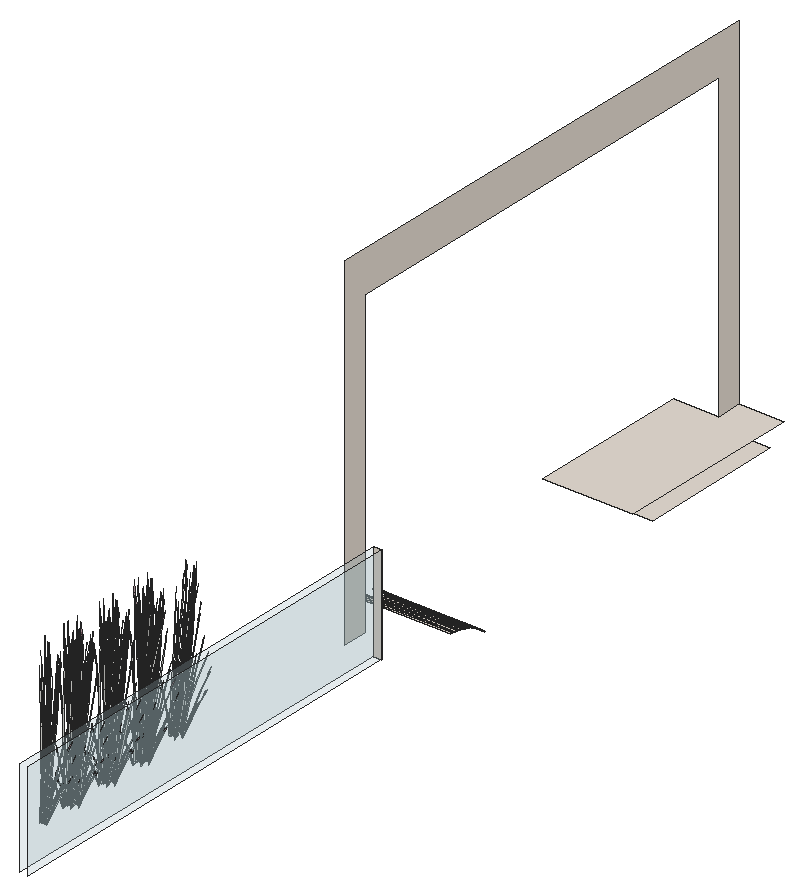
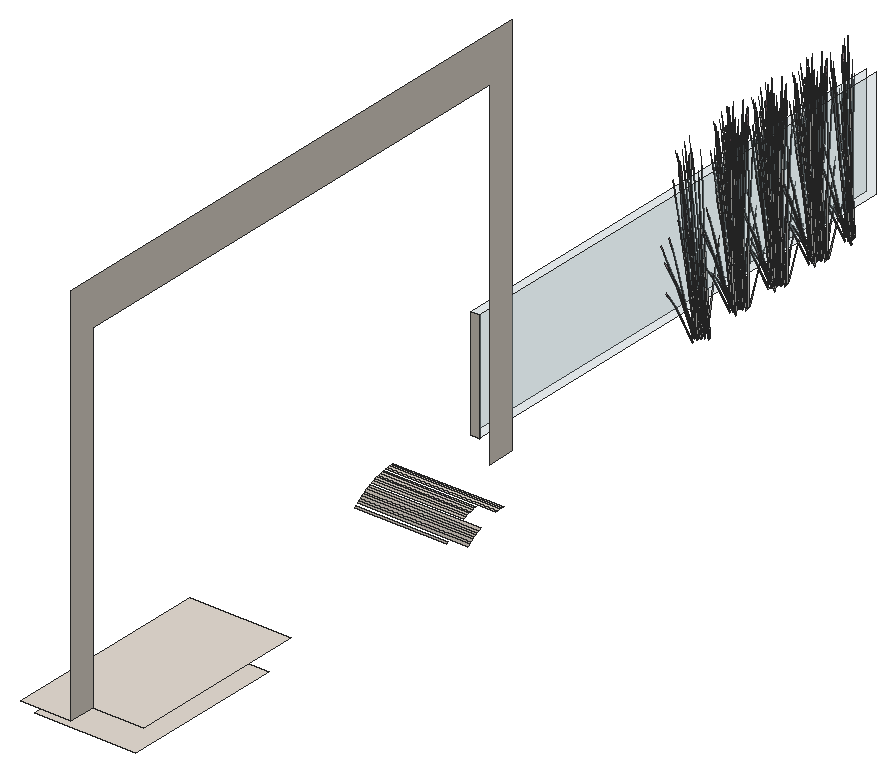
# SketchUp Ruby script. Lengths in inches.
U = 1.inch
M = Sketchup.active_model
def pt(a) = Geom::Point3d.new(a.map { |v| v * U })
def face(e, loops, mat)
  f = e.add_face(loops[0].map { |a| pt(a) })
  loops[1..].each { |l| e.add_face(l.map { |a| pt(a) }).erase! }
  f.material = f.back_material = mat if mat
  f
end
# faces: each face lists its corners as indices into pts; further lists are holes
def faces(e, pts, list, mat = nil) = list.each { |f| face(e, (f[0].is_a?(Array) ? f : [f]).map { |l| l.map { |i| pts[i] } }, mat) }
# xy, xz, yz: faces in a plane at the given z, y or x. An outline is a flat list of corners, or four numbers for a rectangle; further outlines are holes
def ring(l) = l.size == 4 ? [[l[0], l[1]], [l[2], l[1]], [l[2], l[3]], [l[0], l[3]]] : l.each_slice(2).to_a
def flat(e, list, mat, &to3) = list.each { |f| face(e, (f[0].is_a?(Array) ? f : [f]).map { |l| ring(l).map { |u, v| to3.(u, v) } }, mat) }
def xy(e, z, list, mat = nil) = flat(e, list, mat) { |x, y| [x, y, z] }
def xz(e, y, list, mat = nil) = flat(e, list, mat) { |x, z| [x, y, z] }
def yz(e, x, list, mat = nil) = flat(e, list, mat) { |y, z| [x, y, z] }
def lines(e, pts, list) = list.each { |a, b| e.add_line(pt(pts[a]), pt(pts[b])) }
# prism: a flat outline (further loops are holes) pulled along v
def prism(e, loops, v, mat = nil)
  f = face(e, loops, mat); d = Geom::Vector3d.new(v.map { |x| x * U })
  f.pushpull(f.normal.samedirection?(d) ? d.length : -d.length)
end
def box(e, o, s, mat = nil) = prism(e, [[o, [o[0] + s[0], o[1], o[2]], [o[0] + s[0], o[1] + s[1], o[2]], [o[0], o[1] + s[1], o[2]]]], [0, 0, s[2]], mat)
def at(x, y, z, deg = 0) = Geom::Transformation.translation(pt([x, y, z])) * Geom::Transformation.rotation(ORIGIN, Z_AXIS, deg.degrees)
def axes(o, x, y, z) = Geom::Transformation.new([*x, 0, *y, 0, *z, 0, *pt(o).to_a, 1])
def part(name) = M.definitions.add(name)
# library, detail: a bought-in or finely detailed component or shape, given as its bounding box
def library(name, o, s) = part(name).tap { |d| box(d.entities, o, s) }
def detail(e, o, s) = box(e.add_group.entities, o, s)
def put(e, d, t, mat = nil) = e.add_instance(d, t).tap { |i| i.material = mat if mat }
def group(e, t, mat = nil) = e.add_group.tap { |g| g.transformation = t; g.material = mat if mat }.entities
root = M.entities
M.materials.add("Glass_Safety_01").color = [204, 235, 244]
M.materials["Glass_Safety_01"].alpha = 0.25
M.materials.add("LightPink_Translucent").color = [144, 107, 117]
M.materials["LightPink_Translucent"].alpha = 0.75
M.materials.add("Marble_01_1K").color = [230, 221, 211]
c1 = part("blade")
p = [[2.15,0.21,22],[0,0.17,0],[0.09,0.45,0],[2.18,0.31,22],[2.29,0.31,22],[0.38,0.45,0],
  [2.48,0.24,33],[2.49,0.24,33],[2.48,0.22,33]]
faces(c1.entities,p,[[0,1,2,3],[4,5,2,3],[6,3,4,7],[8,0,3,6]])
c2 = part("seeds")
p = [[0.3,-0.1,1.38],[-0.01,-0.03,1.59],[-0.01,-0.03,0.03],[0.14,-0.07,-0.07],[0.29,-0.03,3],[0.15,0.01,3.11]]
faces(c2.entities,p,[[0,1,2,3],[1,0,4,5]],"LightPink_Translucent")
c3 = part("blade with seeds")
put(c3.entities,c1,at(0,0,0))
put(c3.entities,c2,axes([2.4,0.25,30.99],[1.5799,-0.05474,1.17369],[-0.12525,1.92788,0.29478],[-0.07173,-0.02425,1.56792]))
xy(root,258,[[321,336,354,390]],"Marble_01_1K")
xy(root,264,[[321,327,354,327,354,396,337.5,396,337.5,387,321,387]],"Marble_01_1K")
xz(root,216,[[348,264,351,300]],"Marble_01_1K")
yz(root,337.5,[[216,264,225,264,225,375,387,375,387,264,396,264,396,390,216,390]],"Marble_01_1K")
yz(root,348,[[54.05,264,216,300]],"Glass_Safety_01")
yz(root,351,[[54,264,216,300]],"Glass_Safety_01")
p = [[357,255.125,258.3],[357,255.69,257.81],[327,255.69,257.81],[327,255.125,258.3],[357,253.95,259.22],[357,254.54,258.77],
  [321,254.54,258.77],[321,253.95,259.22],[357,253.34,259.65],[321,253.34,259.65],[357,252.71,260.07],[321,252.71,260.07],
  [357,252.08,260.46],[321,252.08,260.46],[357,251.43,260.84],[321,251.43,260.84],[357,250.77,261.2],[321,250.77,261.2],
  [357,250.11,261.54],[321,250.11,261.54],[357,249.43,261.85],[321,249.43,261.85],[357,248.04,262.42],[357,248.74,262.15],
  [327,248.74,262.15],[327,248.04,262.42],[357,247.34,262.68],[327,247.34,262.68],[357,246.625,262.91],[327,246.625,262.91],
  [357,245.91,263.12],[327,245.91,263.12],[357,245.18,263.31],[327,245.18,263.31],[357,244.45,263.47],[327,244.45,263.47],
  [357,243.72,263.62],[327,243.72,263.62],[357,242.24,263.84],[357,242.98,263.74],[321,242.98,263.74],[321,242.24,263.84],
  [357,241.49,263.91],[321,241.49,263.91],[357,240.75,263.97],[321,240.75,263.97],[357,240,264],[321,240,264]]
faces(root,p,[[0,1,2,3],[4,5,6,7],[8,4,7,9],[10,8,9,11],[12,10,11,13],[14,12,13,15],[16,14,15,17],[18,16,17,19],
  [20,18,19,21],[22,23,24,25],[26,22,25,27],[28,26,27,29],[30,28,29,31],[32,30,31,33],[34,32,33,35],[36,34,35,37],
  [38,39,40,41],[42,38,41,43],[44,42,43,45],[46,44,45,47]],"Marble_01_1K")
put(root,c3,axes([336.35,109.73,266.4375],[0.37783,0.32657,0.13483],[-0.31516,0.36844,-0.38503],[-0.08772,0.04981,1.18024]))
put(root,c3,axes([336.35,93.3125,266.4375],[0.37783,0.32657,0.13483],[-0.31516,0.36844,-0.38503],[-0.08772,0.04981,1.18024]))
put(root,c3,axes([336.35,78.43,266.4375],[0.37783,0.32657,0.13483],[-0.31516,0.36844,-0.38503],[-0.08772,0.04981,1.18024]))
put(root,c3,axes([336.21,125.17,266.14],[-0.47569,-0.46784,-0.05709],[0.47598,-0.46812,0],[-0.01661,-0.01634,1.63492]))
put(root,c3,axes([336.21,109.33,266.14],[-0.47569,-0.46784,-0.05709],[0.47598,-0.46812,0],[-0.01661,-0.01634,1.63492]))
put(root,c3,axes([336.21,92.91,266.14],[-0.47569,-0.46784,-0.05709],[0.47598,-0.46812,0],[-0.01661,-0.01634,1.63492]))
put(root,c3,axes([336.34,125.33,266.53],[0.55535,-0.03355,0.41661],[0.05022,0.55698,-0.2005],[-0.09942,0.05645,1.33761]))
put(root,c3,axes([336.34,109.49,266.53],[0.55535,-0.03355,0.41661],[0.05022,0.55698,-0.2005],[-0.09942,0.05645,1.33761]))
put(root,c3,axes([336.34,93.07,266.53],[0.55535,-0.03355,0.41661],[0.05022,0.55698,-0.2005],[-0.09942,0.05645,1.33761]))
put(root,c3,axes([336.34,78.1875,266.53],[0.55535,-0.03355,0.41661],[0.05022,0.55698,-0.2005],[-0.09942,0.05645,1.33761]))
put(root,c3,axes([334.31,142.81,266.48],[0.57594,0.25935,-0.27094],[-0.27732,0.5474,-0.46562],[0.0181,0.1344,1.4872]))
put(root,c3,axes([336.47,126.61,266.17],[0.64025,0.17667,0.2864],[-0.16018,0.63149,-0.33981],[-0.10597,0.07904,1.53541]))
put(root,c3,axes([336.47,110.77,266.17],[0.64025,0.17667,0.2864],[-0.16018,0.63149,-0.33981],[-0.10597,0.07904,1.53541]))
put(root,c3,axes([336.47,94.35,266.17],[0.64025,0.17667,0.2864],[-0.16018,0.63149,-0.33981],[-0.10597,0.07904,1.53541]))
put(root,c3,axes([336.47,79.47,266.17],[0.64025,0.17667,0.2864],[-0.16018,0.63149,-0.33981],[-0.10597,0.07904,1.53541]))
put(root,c3,axes([335.54,121.77,265.39],[-0.08578,0.01958,1.6421],[-0.47437,-0.22044,-0.25086],[0.00796,-0.18387,0.2797]))
put(root,c3,axes([335.54,105.93,265.39],[-0.08578,0.01958,1.6421],[-0.47437,-0.22044,-0.25086],[0.00796,-0.18387,0.2797]))
put(root,c3,axes([335.54,89.51,265.39],[-0.08578,0.01958,1.6421],[-0.47437,-0.22044,-0.25086],[0.00796,-0.18387,0.2797]))
put(root,c3,axes([333.08,140.95,265.89],[0.47712,0.13449,-0.28847],[-0.12013,0.47362,0.28847],[0.09619,-0.05462,1.29413]))
put(root,c3,axes([336.75,126.58,266.31],[0.47863,-0.27177,0.46235],[0.28609,0.48733,0],[-0.10901,0.0619,1.46668]))
put(root,c3,axes([336.75,110.74,266.31],[0.47863,-0.27177,0.46235],[0.28609,0.48733,0],[-0.10901,0.0619,1.46668]))
put(root,c3,axes([336.75,94.32,266.31],[0.47863,-0.27177,0.46235],[0.28609,0.48733,0],[-0.10901,0.0619,1.46668]))
put(root,c3,axes([336.75,79.43,266.31],[0.47863,-0.27177,0.46235],[0.28609,0.48733,0],[-0.10901,0.0619,1.46668]))
put(root,c3,axes([334.41,140.375,266.41],[-0.14537,0.11002,1.33163],[-0.43536,-0.19256,-0.28638],[0.0807,-0.23948,0.56934]))
put(root,c3,axes([335.25,124.63,266.2],[0.22235,0.6078,0.42607],[-0.63531,0.21135,0.16719],[0.00776,-0.11168,1.47927]))
put(root,c3,axes([335.25,108.79,266.2],[0.22235,0.6078,0.42607],[-0.63531,0.21135,0.16719],[0.00776,-0.11168,1.47927]))
put(root,c3,axes([335.25,92.37,266.2],[0.22235,0.6078,0.42607],[-0.63531,0.21135,0.16719],[0.00776,-0.11168,1.47927]))
put(root,c3,axes([335.15,124.55,266.06],[0.24813,-0.48978,-0.41661],[0.51557,0.23571,0.2005],[0,-0.1129,1.33761]))
put(root,c3,axes([335.15,108.71,266.06],[0.24813,-0.48978,-0.41661],[0.51557,0.23571,0.2005],[0,-0.1129,1.33761]))
put(root,c3,axes([335.15,92.29,266.06],[0.24813,-0.48978,-0.41661],[0.51557,0.23571,0.2005],[0,-0.1129,1.33761]))
put(root,c3,axes([335.79,126.13,266.05],[-0.16686,-0.46861,0],[0.47648,-0.16411,0],[0,0,1.4375]))
put(root,c3,axes([335.79,110.29,266.05],[-0.16686,-0.46861,0],[0.47648,-0.16411,0],[0,0,1.4375]))
put(root,c3,axes([335.79,93.875,266.05],[-0.16686,-0.46861,0],[0.47648,-0.16411,0],[0,0,1.4375]))
put(root,c3,axes([335.18,127.12,265.39],[0.08277,-0.02958,1.6421],[0.49786,0.16279,-0.25086],[0.01456,0.18348,0.2797]))
put(root,c3,axes([335.18,111.28,265.39],[0.08277,-0.02958,1.6421],[0.49786,0.16279,-0.25086],[0.01456,0.18348,0.2797]))
put(root,c3,axes([335.18,94.86,265.39],[0.08277,-0.02958,1.6421],[0.49786,0.16279,-0.25086],[0.01456,0.18348,0.2797]))
put(root,c3,axes([335.18,79.98,265.39],[0.08277,-0.02958,1.6421],[0.49786,0.16279,-0.25086],[0.01456,0.18348,0.2797]))
put(root,c3,axes([335.56,142.93,266.31],[0,-0.54355,0.46235],[0.57217,0,0],[0,0.1238,1.46668]))
put(root,c3,axes([335.8,143.4375,265.88],[0,0.54355,-0.46235],[-0.57217,0,0],[0,0.1238,1.46668]))
put(root,c3,axes([332.97,140.73,265.88],[0.47863,-0.27177,-0.46235],[0.28609,0.48733,0],[0.10901,-0.0619,1.46668]))
put(root,c3,axes([333.93,142.08,266.4375],[0.09866,-0.48509,0.13483],[0.48202,0.0842,-0.38503],[0.08772,0.04981,1.18024]))
put(root,c3,axes([334.61,141.24,266.31],[-0.47863,-0.27177,0.46235],[0.28609,-0.48733,0],[0.10901,0.0619,1.46668]))
put(root,c3,axes([336.46,125.21,266.06],[-0.24813,0.48978,-0.41661],[-0.51557,-0.23571,0.2005],[0,0.1129,1.33761]))
put(root,c3,axes([336.46,109.37,266.06],[-0.24813,0.48978,-0.41661],[-0.51557,-0.23571,0.2005],[0,0.1129,1.33761]))
put(root,c3,axes([336.46,92.95,266.06],[-0.24813,0.48978,-0.41661],[-0.51557,-0.23571,0.2005],[0,0.1129,1.33761]))
put(root,c3,axes([336.46,78.0625,266.06],[-0.24813,0.48978,-0.41661],[-0.51557,-0.23571,0.2005],[0,0.1129,1.33761]))
put(root,c3,axes([334.2,144.07,266.03],[0.53691,-0.18442,-0.17877],[0.18866,0.53125,0.00007],[0.05927,-0.02038,1.61933]))
put(root,c3,axes([337.44,124.91,266.3],[-0.40181,-0.39593,0.16428],[0.40492,-0.38402,0.32672],[-0.04438,0.08086,1.49371]))
put(root,c3,axes([337.44,109.07,266.3],[-0.40181,-0.39593,0.16428],[0.40492,-0.38402,0.32672],[-0.04438,0.08086,1.49371]))
put(root,c3,axes([337.44,92.65,266.3],[-0.40181,-0.39593,0.16428],[0.40492,-0.38402,0.32672],[-0.04438,0.08086,1.49371]))
put(root,c3,axes([336.05,124.68,266.05],[0,-0.62892,0],[0.63949,0,0],[0,0,1.6711]))
put(root,c3,axes([336.05,108.84,266.05],[0,-0.62892,0],[0.63949,0,0],[0,0,1.6711]))
put(root,c3,axes([336.05,92.42,266.05],[0,-0.62892,0],[0.63949,0,0],[0,0,1.6711]))
put(root,c3,axes([335.46,124.79,266.27],[0.57623,0.26344,0.22409],[-0.27732,0.5474,0.46562],[0,-0.12618,1.49497]))
put(root,c3,axes([335.46,108.96,266.27],[0.57623,0.26344,0.22409],[-0.27732,0.5474,0.46562],[0,-0.12618,1.49497]))
put(root,c3,axes([335.46,92.54,266.27],[0.57623,0.26344,0.22409],[-0.27732,0.5474,0.46562],[0,-0.12618,1.49497]))
put(root,c3,axes([336.375,124.93,266.13],[0,0.62861,-0.05249],[-0.63949,0,0],[0,0.01975,1.67027]))
put(root,c3,axes([336.375,109.09,266.13],[0,0.62861,-0.05249],[-0.63949,0,0],[0,0.01975,1.67027]))
put(root,c3,axes([336.375,92.67,266.13],[0,0.62861,-0.05249],[-0.63949,0,0],[0,0.01975,1.67027]))
put(root,c3,axes([336.375,77.79,266.13],[0,0.62861,-0.05249],[-0.63949,0,0],[0,0.01975,1.67027]))
put(root,c3,axes([335.27,124.43,266.53],[-0.55535,0.03355,0.41661],[-0.05022,-0.55698,-0.2005],[0.09942,-0.05645,1.33761]))
put(root,c3,axes([335.27,108.59,266.53],[-0.55535,0.03355,0.41661],[-0.05022,-0.55698,-0.2005],[0.09942,-0.05645,1.33761]))
put(root,c3,axes([335.27,92.17,266.53],[-0.55535,0.03355,0.41661],[-0.05022,-0.55698,-0.2005],[0.09942,-0.05645,1.33761]))
put(root,c3,axes([334.21,142.5,266.06],[0.30722,0.45622,-0.41661],[-0.46535,0.32126,0.2005],[0.09942,0.05645,1.33761]))
put(root,c3,axes([335.02,123.47,266.3],[-0.14774,0.54019,0.16428],[-0.54062,-0.15287,0.32672],[0.09339,-0.00263,1.49371]))
put(root,c3,axes([335.02,107.63,266.3],[-0.14774,0.54019,0.16428],[-0.54062,-0.15287,0.32672],[0.09339,-0.00263,1.49371]))
put(root,c3,axes([335.02,91.21,266.3],[-0.14774,0.54019,0.16428],[-0.54062,-0.15287,0.32672],[0.09339,-0.00263,1.49371]))
put(root,c3,axes([336.07,126.15,266.13],[0.22235,0.62444,-0.05599],[-0.63531,0.21881,0],[0.00776,0.02181,1.60327]))
put(root,c3,axes([336.07,110.31,266.13],[0.22235,0.62444,-0.05599],[-0.63531,0.21881,0],[0.00776,0.02181,1.60327]))
put(root,c3,axes([336.07,93.89,266.13],[0.22235,0.62444,-0.05599],[-0.63531,0.21881,0],[0.00776,0.02181,1.60327]))
put(root,c3,axes([336.07,79,266.13],[0.22235,0.62444,-0.05599],[-0.63531,0.21881,0],[0.00776,0.02181,1.60327]))
put(root,c3,axes([334.05,144.4,266.41],[0.00902,-0.18018,1.33163],[0.43127,-0.20126,-0.28638],[0.13313,0.21566,0.56934]))
put(root,c3,axes([334.75,122.81,266.21],[-0.31974,-0.54466,0],[0.53494,-0.30375,-0.48057],[0.12184,-0.06918,1.52448]))
put(root,c3,axes([334.75,106.97,266.21],[-0.31974,-0.54466,0],[0.53494,-0.30375,-0.48057],[0.12184,-0.06918,1.52448]))
put(root,c3,axes([334.75,90.55,266.21],[-0.31974,-0.54466,0],[0.53494,-0.30375,-0.48057],[0.12184,-0.06918,1.52448]))
put(root,c3,axes([337.91,125.33,266.05],[-0.63917,-0.00435,-0.04634],[0,-0.60749,0.46507],[-0.02009,0.13829,1.47457]))
put(root,c3,axes([337.91,109.49,266.05],[-0.63917,-0.00435,-0.04634],[0,-0.60749,0.46507],[-0.02009,0.13829,1.47457]))
put(root,c3,axes([337.91,93.07,266.05],[-0.63917,-0.00435,-0.04634],[0,-0.60749,0.46507],[-0.02009,0.13829,1.47457]))
put(root,c3,axes([337.91,78.18,266.05],[-0.63917,-0.00435,-0.04634],[0,-0.60749,0.46507],[-0.02009,0.13829,1.47457]))
put(root,c3,axes([333.54,141.85,265.92],[0.34446,-0.40855,-0.58063],[0.42791,0.37046,-0.15239],[0.13803,-0.10191,1.28164]))
put(root,c3,axes([336.65,123.5,266.3],[-0.54955,0.14427,0.16428],[-0.1357,-0.53689,0.32672],[0.04901,0.07823,1.49371]))
put(root,c3,axes([336.65,107.66,266.3],[-0.54955,0.14427,0.16428],[-0.1357,-0.53689,0.32672],[0.04901,0.07823,1.49371]))
put(root,c3,axes([336.65,91.24,266.3],[-0.54955,0.14427,0.16428],[-0.1357,-0.53689,0.32672],[0.04901,0.07823,1.49371]))
put(root,c3,axes([336.09,105.65,266.58],[0.06561,0.31695,1.06958],[-0.36394,-0.17555,0.78586],[0.03916,-0.16229,0.23558]))
put(root,c3,axes([336.09,89.23,266.58],[0.06561,0.31695,1.06958],[-0.36394,-0.17555,0.78586],[0.03916,-0.16229,0.23558]))
put(root,c3,axes([335.05,141.48,265.89],[0.12013,0.47362,-0.28847],[-0.47712,0.13449,0.28847],[0.09619,0.05462,1.29413]))
put(root,c3,axes([335.95,143.03,266.21],[0.63949,0,0],[0,0.60749,-0.48057],[0,0.13836,1.52448]))
put(root,c3,axes([335.75,124.28,266.2],[-0.42403,0.49328,0.42607],[-0.50377,-0.43543,0.16719],[0.10223,-0.04923,1.47927]))
put(root,c3,axes([335.75,108.44,266.2],[-0.42403,0.49328,0.42607],[-0.50377,-0.43543,0.16719],[0.10223,-0.04923,1.47927]))
put(root,c3,axes([335.75,92.03,266.2],[-0.42403,0.49328,0.42607],[-0.50377,-0.43543,0.16719],[0.10223,-0.04923,1.47927]))
put(root,c3,axes([336.48,125.0625,266.0625],[0.35699,0.35109,0],[-0.35699,0.35109,0],[0,0,1.57621]))
put(root,c3,axes([336.48,109.22,266.0625],[0.35699,0.35109,0],[-0.35699,0.35109,0],[0,0,1.57621]))
put(root,c3,axes([336.48,92.8,266.0625],[0.35699,0.35109,0],[-0.35699,0.35109,0],[0,0,1.57621]))
put(root,c3,axes([336.47,124.65,266.53],[0.24813,-0.48978,0.41661],[0.51557,0.23571,-0.2005],[0,0.1129,1.33761]))
put(root,c3,axes([336.47,108.8125,266.53],[0.24813,-0.48978,0.41661],[0.51557,0.23571,-0.2005],[0,0.1129,1.33761]))
put(root,c3,axes([336.47,92.39,266.53],[0.24813,-0.48978,0.41661],[0.51557,0.23571,-0.2005],[0,0.1129,1.33761]))
put(root,c3,axes([336.47,77.51,266.53],[0.24813,-0.48978,0.41661],[0.51557,0.23571,-0.2005],[0,0.1129,1.33761]))
put(root,c3,axes([336.26,126.35,266.05],[0.51557,0.24403,0],[-0.24813,0.50705,0],[0,0,1.62917]))
put(root,c3,axes([336.26,110.51,266.05],[0.51557,0.24403,0],[-0.24813,0.50705,0],[0,0,1.62917]))
put(root,c3,axes([336.26,94.09,266.05],[0.51557,0.24403,0],[-0.24813,0.50705,0],[0,0,1.62917]))
put(root,c3,axes([336.26,79.21,266.05],[0.51557,0.24403,0],[-0.24813,0.50705,0],[0,0,1.62917]))
put(root,c3,axes([333.88,142.24,266.48],[0.51635,-0.36087,-0.27094],[0.34336,0.5099,-0.46562],[0.1274,0.05178,1.4872]))
put(root,c3,axes([335.12,145.28,266.48],[-0.32795,-0.01705,0.97832],[0.21658,-0.36206,0.54015],[0.12956,0.12863,0.76741]))
put(root,c3,axes([336.3,124.53,266.22],[-0.64638,-0.11452,0.45814],[0.13155,-0.64678,0.17978],[0.09446,0.06245,1.59061]))
put(root,c3,axes([336.3,108.69,266.22],[-0.64638,-0.11452,0.45814],[0.13155,-0.64678,0.17978],[0.09446,0.06245,1.59061]))
put(root,c3,axes([336.3,92.28,266.22],[-0.64638,-0.11452,0.45814],[0.13155,-0.64678,0.17978],[0.09446,0.06245,1.59061]))
put(root,c3,axes([337.77,125.42,265.89],[-0.35699,0.33913,-0.28847],[-0.35699,-0.33913,0.28847],[0,0.10923,1.29413]))
put(root,c3,axes([337.77,109.58,265.89],[-0.35699,0.33913,-0.28847],[-0.35699,-0.33913,0.28847],[0,0.10923,1.29413]))
put(root,c3,axes([337.77,93.16,265.89],[-0.35699,0.33913,-0.28847],[-0.35699,-0.33913,0.28847],[0,0.10923,1.29413]))
put(root,c3,axes([337.77,78.27,265.89],[-0.35699,0.33913,-0.28847],[-0.35699,-0.33913,0.28847],[0,0.10923,1.29413]))
put(root,c3,axes([336.75,125.35,265.95],[0.18752,0.49766,-0.6445],[-0.54017,0.17923,-0.16915],[0.02073,0.16852,1.42262]))
put(root,c3,axes([336.75,109.52,265.95],[0.18752,0.49766,-0.6445],[-0.54017,0.17923,-0.16915],[0.02073,0.16852,1.42262]))
put(root,c3,axes([336.75,93.1,265.95],[0.18752,0.49766,-0.6445],[-0.54017,0.17923,-0.16915],[0.02073,0.16852,1.42262]))
put(root,c3,axes([336.75,78.21,265.95],[0.18752,0.49766,-0.6445],[-0.54017,0.17923,-0.16915],[0.02073,0.16852,1.42262]))
put(root,c3,axes([336.49,124.82,266.05],[0.57217,0,0],[0,0.56272,0],[0,0,1.66132]))
put(root,c3,axes([336.49,108.98,266.05],[0.57217,0,0],[0,0.56272,0],[0,0,1.66132]))
put(root,c3,axes([336.49,92.5625,266.05],[0.57217,0,0],[0,0.56272,0],[0,0,1.66132]))
put(root,c3,axes([335.9375,124.2,266.53],[-0.30722,-0.45622,0.41661],[0.46535,-0.32126,-0.2005],[0.09942,0.05645,1.33761]))
put(root,c3,axes([335.9375,108.36,266.53],[-0.30722,-0.45622,0.41661],[0.46535,-0.32126,-0.2005],[0.09942,0.05645,1.33761]))
put(root,c3,axes([335.9375,91.94,266.53],[-0.30722,-0.45622,0.41661],[0.46535,-0.32126,-0.2005],[0.09942,0.05645,1.33761]))
put(root,c3,axes([335.38,124.31,266.48],[-0.05959,-0.62022,-0.27094],[0.62068,-0.0375,-0.46562],[0.1093,-0.08261,1.4872]))
put(root,c3,axes([335.38,108.47,266.48],[-0.05959,-0.62022,-0.27094],[0.62068,-0.0375,-0.46562],[0.1093,-0.08261,1.4872]))
put(root,c3,axes([335.38,92.05,266.48],[-0.05959,-0.62022,-0.27094],[0.62068,-0.0375,-0.46562],[0.1093,-0.08261,1.4872]))
put(root,c3,axes([336.6875,124.76,266.4375],[0.47648,-0.15851,0.13483],[0.16686,0.45265,-0.38503],[0,0.09962,1.18024]))
put(root,c3,axes([336.6875,108.92,266.4375],[0.47648,-0.15851,0.13483],[0.16686,0.45265,-0.38503],[0,0.09962,1.18024]))
put(root,c3,axes([336.6875,92.51,266.4375],[0.47648,-0.15851,0.13483],[0.16686,0.45265,-0.38503],[0,0.09962,1.18024]))
put(root,c3,axes([336.6875,77.62,266.4375],[0.47648,-0.15851,0.13483],[0.16686,0.45265,-0.38503],[0,0.09962,1.18024]))
put(root,c3,axes([332.58,141.92,265.48],[-0.50338,0.21762,1.20058],[-0.16022,-0.62439,0.4665],[0.30911,0.01039,1.36553]))
put(root,c3,axes([336.52,124.8,266.48],[0.57594,0.25935,-0.27094],[-0.27732,0.5474,-0.46562],[0.0181,0.1344,1.4872]))
put(root,c3,axes([336.52,108.96,266.48],[0.57594,0.25935,-0.27094],[-0.27732,0.5474,-0.46562],[0.0181,0.1344,1.4872]))
put(root,c3,axes([336.52,92.54,266.48],[0.57594,0.25935,-0.27094],[-0.27732,0.5474,-0.46562],[0.0181,0.1344,1.4872]))
put(root,c3,axes([336.52,77.66,266.48],[0.57594,0.25935,-0.27094],[-0.27732,0.5474,-0.46562],[0.0181,0.1344,1.4872]))
put(root,c3,axes([334.89,140.95,266.21],[0.31974,-0.54466,0],[0.53494,0.30375,-0.48057],[0.12184,0.06918,1.52448]))
put(root,c3,axes([335.43,140.71,265.39],[-0.07655,-0.04282,1.6421],[-0.19662,-0.47839,-0.25086],[0.13264,-0.12982,0.2797]))
put(root,c3,axes([335.3,122.9375,265.89],[0.47712,0.13449,-0.28847],[-0.12013,0.47362,0.28847],[0.09619,-0.05462,1.29413]))
put(root,c3,axes([335.3,107.1,265.89],[0.47712,0.13449,-0.28847],[-0.12013,0.47362,0.28847],[0.09619,-0.05462,1.29413]))
put(root,c3,axes([335.3,90.68,265.89],[0.47712,0.13449,-0.28847],[-0.12013,0.47362,0.28847],[0.09619,-0.05462,1.29413]))
put(root,c3,axes([336.625,122.36,266.41],[-0.14537,0.11002,1.33163],[-0.43536,-0.19256,-0.28638],[0.0807,-0.23948,0.56934]))
put(root,c3,axes([336.625,106.53,266.41],[-0.14537,0.11002,1.33163],[-0.43536,-0.19256,-0.28638],[0.0807,-0.23948,0.56934]))
put(root,c3,axes([336.625,90.11,266.41],[-0.14537,0.11002,1.33163],[-0.43536,-0.19256,-0.28638],[0.0807,-0.23948,0.56934]))
put(root,c3,axes([335.18,141.28,265.88],[0.47863,0.27177,-0.46235],[-0.28609,0.48733,0],[0.10901,0.0619,1.46668]))
put(root,c3,axes([335.16,145.15,265.39],[0.03726,-0.07847,1.6421],[0.46909,-0.23111,-0.25086],[0.14221,0.11962,0.2797]))
put(root,c3,axes([337.77,124.92,266.31],[0,-0.54355,0.46235],[0.57217,0,0],[0,0.1238,1.46668]))
put(root,c3,axes([337.77,109.08,266.31],[0,-0.54355,0.46235],[0.57217,0,0],[0,0.1238,1.46668]))
put(root,c3,axes([337.77,92.67,266.31],[0,-0.54355,0.46235],[0.57217,0,0],[0,0.1238,1.46668]))
put(root,c3,axes([337.77,77.78,266.31],[0,-0.54355,0.46235],[0.57217,0,0],[0,0.1238,1.46668]))
put(root,c3,axes([338.02,125.43,265.88],[0,0.54355,-0.46235],[-0.57217,0,0],[0,0.1238,1.46668]))
put(root,c3,axes([338.02,109.59,265.88],[0,0.54355,-0.46235],[-0.57217,0,0],[0,0.1238,1.46668]))
put(root,c3,axes([338.02,93.17,265.88],[0,0.54355,-0.46235],[-0.57217,0,0],[0,0.1238,1.46668]))
put(root,c3,axes([338.02,78.28,265.88],[0,0.54355,-0.46235],[-0.57217,0,0],[0,0.1238,1.46668]))
put(root,c3,axes([335.18,122.72,265.88],[0.47863,-0.27177,-0.46235],[0.28609,0.48733,0],[0.10901,-0.0619,1.46668]))
put(root,c3,axes([335.18,106.88,265.88],[0.47863,-0.27177,-0.46235],[0.28609,0.48733,0],[0.10901,-0.0619,1.46668]))
put(root,c3,axes([335.18,90.46,265.88],[0.47863,-0.27177,-0.46235],[0.28609,0.48733,0],[0.10901,-0.0619,1.46668]))
put(root,c3,axes([336.14,124.07,266.4375],[0.09866,-0.48509,0.13483],[0.48202,0.0842,-0.38503],[0.08772,0.04981,1.18024]))
put(root,c3,axes([336.14,108.23,266.4375],[0.09866,-0.48509,0.13483],[0.48202,0.0842,-0.38503],[0.08772,0.04981,1.18024]))
put(root,c3,axes([336.14,91.81,266.4375],[0.09866,-0.48509,0.13483],[0.48202,0.0842,-0.38503],[0.08772,0.04981,1.18024]))
put(root,c3,axes([334.48,142.32,265.92],[0.53199,0.08911,-0.58063],[-0.11226,0.54969,-0.15239],[0.15876,0.06661,1.28164]))
put(root,c3,axes([336.75,142.64,266.11],[-0.31706,-0.34757,-0.06041],[0.34725,-0.31847,-0.27392],[0.09839,-0.02242,0.90349]))
put(root,c3,axes([336.83,123.23,266.31],[-0.47863,-0.27177,0.46235],[0.28609,-0.48733,0],[0.10901,0.0619,1.46668]))
put(root,c3,axes([336.83,107.39,266.31],[-0.47863,-0.27177,0.46235],[0.28609,-0.48733,0],[0.10901,0.0619,1.46668]))
put(root,c3,axes([336.83,90.97,266.31],[-0.47863,-0.27177,0.46235],[0.28609,-0.48733,0],[0.10901,0.0619,1.46668]))
put(root,c3,axes([336.41,126.07,266.03],[0.53691,-0.18442,-0.17877],[0.18866,0.53125,0.00007],[0.05927,-0.02038,1.61933]))
put(root,c3,axes([336.41,110.23,266.03],[0.53691,-0.18442,-0.17877],[0.18866,0.53125,0.00007],[0.05927,-0.02038,1.61933]))
put(root,c3,axes([336.41,93.81,266.03],[0.53691,-0.18442,-0.17877],[0.18866,0.53125,0.00007],[0.05927,-0.02038,1.61933]))
put(root,c3,axes([336.42,124.49,266.06],[0.30722,0.45622,-0.41661],[-0.46535,0.32126,0.2005],[0.09942,0.05645,1.33761]))
put(root,c3,axes([336.42,108.65,266.06],[0.30722,0.45622,-0.41661],[-0.46535,0.32126,0.2005],[0.09942,0.05645,1.33761]))
put(root,c3,axes([336.42,92.23,266.06],[0.30722,0.45622,-0.41661],[-0.46535,0.32126,0.2005],[0.09942,0.05645,1.33761]))
put(root,c3,axes([336.42,77.34,266.06],[0.30722,0.45622,-0.41661],[-0.46535,0.32126,0.2005],[0.09942,0.05645,1.33761]))
put(root,c3,axes([337.29,126.56,266.58],[-0.28795,-0.15629,1.06958],[0.37181,-0.1588,0.78586],[0.10029,0.13452,0.23558]))
put(root,c3,axes([337.29,110.72,266.58],[-0.28795,-0.15629,1.06958],[0.37181,-0.1588,0.78586],[0.10029,0.13452,0.23558]))
put(root,c3,axes([337.29,94.3,266.58],[-0.28795,-0.15629,1.06958],[0.37181,-0.1588,0.78586],[0.10029,0.13452,0.23558]))
put(root,c3,axes([337.29,79.41,266.58],[-0.28795,-0.15629,1.06958],[0.37181,-0.1588,0.78586],[0.10029,0.13452,0.23558]))
put(root,c3,axes([336.27,126.39,266.41],[0.00902,-0.18018,1.33163],[0.43127,-0.20126,-0.28638],[0.13313,0.21566,0.56934]))
put(root,c3,axes([336.27,110.55,266.41],[0.00902,-0.18018,1.33163],[0.43127,-0.20126,-0.28638],[0.13313,0.21566,0.56934]))
put(root,c3,axes([336.27,94.13,266.41],[0.00902,-0.18018,1.33163],[0.43127,-0.20126,-0.28638],[0.13313,0.21566,0.56934]))
put(root,c3,axes([336.27,79.25,266.41],[0.00902,-0.18018,1.33163],[0.43127,-0.20126,-0.28638],[0.13313,0.21566,0.56934]))
put(root,c3,axes([335.75,123.84,265.92],[0.34446,-0.40855,-0.58063],[0.42791,0.37046,-0.15239],[0.13803,-0.10191,1.28164]))
put(root,c3,axes([335.75,108,265.92],[0.34446,-0.40855,-0.58063],[0.42791,0.37046,-0.15239],[0.13803,-0.10191,1.28164]))
put(root,c3,axes([335.75,91.58,265.92],[0.34446,-0.40855,-0.58063],[0.42791,0.37046,-0.15239],[0.13803,-0.10191,1.28164]))
put(root,c3,axes([337.26,123.47,265.89],[0.12013,0.47362,-0.28847],[-0.47712,0.13449,0.28847],[0.09619,0.05462,1.29413]))
put(root,c3,axes([337.26,107.63,265.89],[0.12013,0.47362,-0.28847],[-0.47712,0.13449,0.28847],[0.09619,0.05462,1.29413]))
put(root,c3,axes([337.26,91.22,265.89],[0.12013,0.47362,-0.28847],[-0.47712,0.13449,0.28847],[0.09619,0.05462,1.29413]))
put(root,c3,axes([338.16,125.02,266.21],[0.63949,0,0],[0,0.60749,-0.48057],[0,0.13836,1.52448]))
put(root,c3,axes([338.16,109.18,266.21],[0.63949,0,0],[0,0.60749,-0.48057],[0,0.13836,1.52448]))
put(root,c3,axes([338.16,92.76,266.21],[0.63949,0,0],[0,0.60749,-0.48057],[0,0.13836,1.52448]))
put(root,c3,axes([338.16,77.87,266.21],[0.63949,0,0],[0,0.60749,-0.48057],[0,0.13836,1.52448]))
put(root,c3,axes([336.1,124.23,266.48],[0.51635,-0.36087,-0.27094],[0.34336,0.5099,-0.46562],[0.1274,0.05178,1.4872]))
put(root,c3,axes([336.1,108.39,266.48],[0.51635,-0.36087,-0.27094],[0.34336,0.5099,-0.46562],[0.1274,0.05178,1.4872]))
put(root,c3,axes([336.1,91.97,266.48],[0.51635,-0.36087,-0.27094],[0.34336,0.5099,-0.46562],[0.1274,0.05178,1.4872]))
put(root,c3,axes([337.34,127.27,266.48],[-0.32795,-0.01705,0.97832],[0.21658,-0.36206,0.54015],[0.12956,0.12863,0.76741]))
put(root,c3,axes([337.34,111.43,266.48],[-0.32795,-0.01705,0.97832],[0.21658,-0.36206,0.54015],[0.12956,0.12863,0.76741]))
put(root,c3,axes([337.34,95.01,266.48],[-0.32795,-0.01705,0.97832],[0.21658,-0.36206,0.54015],[0.12956,0.12863,0.76741]))
put(root,c3,axes([337.34,80.125,266.48],[-0.32795,-0.01705,0.97832],[0.21658,-0.36206,0.54015],[0.12956,0.12863,0.76741]))
put(root,c3,axes([335.81,141.67,266.41],[-0.1827,-0.0161,1.33163],[-0.18717,-0.43188,-0.28638],[0.22444,-0.12218,0.56934]))
put(root,c3,axes([334.79,123.91,265.48],[-0.50338,0.21762,1.20058],[-0.16022,-0.62439,0.4665],[0.30911,0.01039,1.36553]))
put(root,c3,axes([334.79,108.07,265.48],[-0.50338,0.21762,1.20058],[-0.16022,-0.62439,0.4665],[0.30911,0.01039,1.36553]))
put(root,c3,axes([334.79,91.65,265.48],[-0.50338,0.21762,1.20058],[-0.16022,-0.62439,0.4665],[0.30911,0.01039,1.36553]))
put(root,c3,axes([336.15,143.1,265.85],[-0.32938,0.06523,1.31842],[-0.05243,-0.51922,0.07547],[0.2307,-0.07859,0.75023]))
put(root,c3,axes([337.11,122.94,266.21],[0.31974,-0.54466,0],[0.53494,0.30375,-0.48057],[0.12184,0.06918,1.52448]))
put(root,c3,axes([337.11,107.1,266.21],[0.31974,-0.54466,0],[0.53494,0.30375,-0.48057],[0.12184,0.06918,1.52448]))
put(root,c3,axes([337.11,90.68,266.21],[0.31974,-0.54466,0],[0.53494,0.30375,-0.48057],[0.12184,0.06918,1.52448]))
put(root,c3,axes([337.64,122.7,265.39],[-0.07655,-0.04282,1.6421],[-0.19662,-0.47839,-0.25086],[0.13264,-0.12982,0.2797]))
put(root,c3,axes([337.64,106.87,265.39],[-0.07655,-0.04282,1.6421],[-0.19662,-0.47839,-0.25086],[0.13264,-0.12982,0.2797]))
put(root,c3,axes([337.64,90.45,265.39],[-0.07655,-0.04282,1.6421],[-0.19662,-0.47839,-0.25086],[0.13264,-0.12982,0.2797]))
put(root,c3,axes([336.51,142.77,265.39],[-0.02673,-0.08252,1.6421],[0.18538,-0.48271,-0.25086],[0.187,-0.00694,0.2797]))
put(root,c3,axes([337.4,123.27,265.88],[0.47863,0.27177,-0.46235],[-0.28609,0.48733,0],[0.10901,0.0619,1.46668]))
put(root,c3,axes([337.4,107.43,265.88],[0.47863,0.27177,-0.46235],[-0.28609,0.48733,0],[0.10901,0.0619,1.46668]))
put(root,c3,axes([337.4,91.01,265.88],[0.47863,0.27177,-0.46235],[-0.28609,0.48733,0],[0.10901,0.0619,1.46668]))
put(root,c3,axes([337.37,127.14,265.39],[0.03726,-0.07847,1.6421],[0.46909,-0.23111,-0.25086],[0.14221,0.11962,0.2797]))
put(root,c3,axes([337.37,111.3,265.39],[0.03726,-0.07847,1.6421],[0.46909,-0.23111,-0.25086],[0.14221,0.11962,0.2797]))
put(root,c3,axes([337.37,94.88,265.39],[0.03726,-0.07847,1.6421],[0.46909,-0.23111,-0.25086],[0.14221,0.11962,0.2797]))
put(root,c3,axes([337.37,79.99,265.39],[0.03726,-0.07847,1.6421],[0.46909,-0.23111,-0.25086],[0.14221,0.11962,0.2797]))
put(root,c3,axes([336.7,124.3125,265.92],[0.53199,0.08911,-0.58063],[-0.11226,0.54969,-0.15239],[0.15876,0.06661,1.28164]))
put(root,c3,axes([336.7,108.47,265.92],[0.53199,0.08911,-0.58063],[-0.11226,0.54969,-0.15239],[0.15876,0.06661,1.28164]))
put(root,c3,axes([336.7,92.05,265.92],[0.53199,0.08911,-0.58063],[-0.11226,0.54969,-0.15239],[0.15876,0.06661,1.28164]))
put(root,c3,axes([338.96,124.63,266.11],[-0.31706,-0.34757,-0.06041],[0.34725,-0.31847,-0.27392],[0.09839,-0.02242,0.90349]))
put(root,c3,axes([338.96,108.8,266.11],[-0.31706,-0.34757,-0.06041],[0.34725,-0.31847,-0.27392],[0.09839,-0.02242,0.90349]))
put(root,c3,axes([338.96,92.38,266.11],[-0.31706,-0.34757,-0.06041],[0.34725,-0.31847,-0.27392],[0.09839,-0.02242,0.90349]))
put(root,c3,axes([338.24,107.03,266.58],[-0.17034,0.27669,1.06958],[-0.14642,-0.37174,0.78586],[0.14069,-0.09315,0.23558]))
put(root,c3,axes([338.24,90.61,266.58],[-0.17034,0.27669,1.06958],[-0.14642,-0.37174,0.78586],[0.14069,-0.09315,0.23558]))
put(root,c3,axes([336.24,143.875,266.41],[-0.12317,-0.13368,1.33163],[0.16025,-0.44223,-0.28638],[0.24919,0.05991,0.56934]))
put(root,c3,axes([339.05,109.43,266.58],[-0.31598,0.08973,1.06958],[0.14873,-0.37085,0.78586],[0.16763,0.02538,0.23558]))
put(root,c3,axes([339.05,93.01,266.58],[-0.31598,0.08973,1.06958],[0.14873,-0.37085,0.78586],[0.16763,0.02538,0.23558]))
put(root,c3,axes([338.03,123.66,266.41],[-0.1827,-0.0161,1.33163],[-0.18717,-0.43188,-0.28638],[0.22444,-0.12218,0.56934]))
put(root,c3,axes([338.03,107.82,266.41],[-0.1827,-0.0161,1.33163],[-0.18717,-0.43188,-0.28638],[0.22444,-0.12218,0.56934]))
put(root,c3,axes([338.03,91.4,266.41],[-0.1827,-0.0161,1.33163],[-0.18717,-0.43188,-0.28638],[0.22444,-0.12218,0.56934]))
put(root,c3,axes([338.36,125.1,265.85],[-0.32938,0.06523,1.31842],[-0.05243,-0.51922,0.07547],[0.2307,-0.07859,0.75023]))
put(root,c3,axes([338.36,109.26,265.85],[-0.32938,0.06523,1.31842],[-0.05243,-0.51922,0.07547],[0.2307,-0.07859,0.75023]))
put(root,c3,axes([338.36,92.84,265.85],[-0.32938,0.06523,1.31842],[-0.05243,-0.51922,0.07547],[0.2307,-0.07859,0.75023]))
put(root,c3,axes([338.72,124.76,265.39],[-0.02673,-0.08252,1.6421],[0.18538,-0.48271,-0.25086],[0.187,-0.00694,0.2797]))
put(root,c3,axes([338.72,108.92,265.39],[-0.02673,-0.08252,1.6421],[0.18538,-0.48271,-0.25086],[0.187,-0.00694,0.2797]))
put(root,c3,axes([338.72,92.5,265.39],[-0.02673,-0.08252,1.6421],[0.18538,-0.48271,-0.25086],[0.187,-0.00694,0.2797]))
put(root,c3,axes([338.46,125.87,266.41],[-0.12317,-0.13368,1.33163],[0.16025,-0.44223,-0.28638],[0.24919,0.05991,0.56934]))
put(root,c3,axes([338.46,110.03,266.41],[-0.12317,-0.13368,1.33163],[0.16025,-0.44223,-0.28638],[0.24919,0.05991,0.56934]))
put(root,c3,axes([338.46,93.61,266.41],[-0.12317,-0.13368,1.33163],[0.16025,-0.44223,-0.28638],[0.24919,0.05991,0.56934]))
put(root,c3,axes([338.46,78.72,266.41],[-0.12317,-0.13368,1.33163],[0.16025,-0.44223,-0.28638],[0.24919,0.05991,0.56934]))
